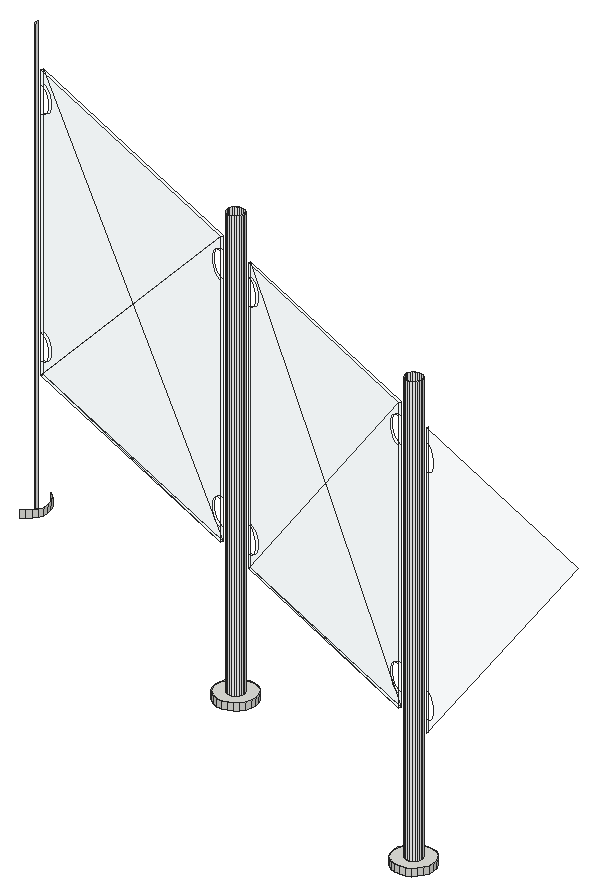
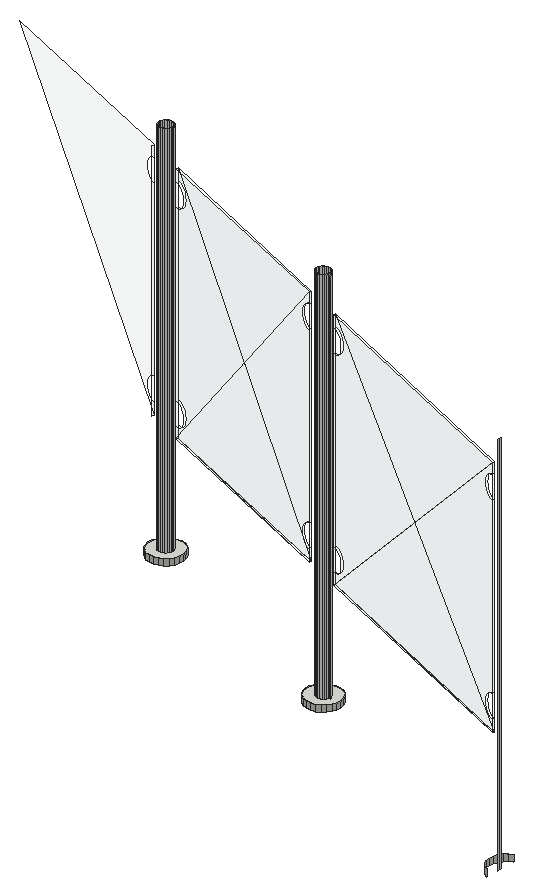
# SketchUp Ruby script. Lengths in inches.
U = 1.inch
M = Sketchup.active_model
def pt(a) = Geom::Point3d.new(a.map { |v| v * U })
def face(e, loops, mat)
  f = e.add_face(loops[0].map { |a| pt(a) })
  loops[1..].each { |l| e.add_face(l.map { |a| pt(a) }).erase! }
  f.material = f.back_material = mat if mat
  f
end
# faces: each face lists its corners as indices into pts; further lists are holes
def faces(e, pts, list, mat = nil) = list.each { |f| face(e, (f[0].is_a?(Array) ? f : [f]).map { |l| l.map { |i| pts[i] } }, mat) }
# xy, xz, yz: faces in a plane at the given z, y or x. An outline is a flat list of corners, or four numbers for a rectangle; further outlines are holes
def ring(l) = l.size == 4 ? [[l[0], l[1]], [l[2], l[1]], [l[2], l[3]], [l[0], l[3]]] : l.each_slice(2).to_a
def flat(e, list, mat, &to3) = list.each { |f| face(e, (f[0].is_a?(Array) ? f : [f]).map { |l| ring(l).map { |u, v| to3.(u, v) } }, mat) }
def xy(e, z, list, mat = nil) = flat(e, list, mat) { |x, y| [x, y, z] }
def xz(e, y, list, mat = nil) = flat(e, list, mat) { |x, z| [x, y, z] }
def yz(e, x, list, mat = nil) = flat(e, list, mat) { |y, z| [x, y, z] }
def lines(e, pts, list) = list.each { |a, b| e.add_line(pt(pts[a]), pt(pts[b])) }
# prism: a flat outline (further loops are holes) pulled along v
def prism(e, loops, v, mat = nil)
  f = face(e, loops, mat); d = Geom::Vector3d.new(v.map { |x| x * U })
  f.pushpull(f.normal.samedirection?(d) ? d.length : -d.length)
end
def box(e, o, s, mat = nil) = prism(e, [[o, [o[0] + s[0], o[1], o[2]], [o[0] + s[0], o[1] + s[1], o[2]], [o[0], o[1] + s[1], o[2]]]], [0, 0, s[2]], mat)
def at(x, y, z, deg = 0) = Geom::Transformation.translation(pt([x, y, z])) * Geom::Transformation.rotation(ORIGIN, Z_AXIS, deg.degrees)
def axes(o, x, y, z) = Geom::Transformation.new([*x, 0, *y, 0, *z, 0, *pt(o).to_a, 1])
def part(name) = M.definitions.add(name)
# library, detail: a bought-in or finely detailed component or shape, given as its bounding box
def library(name, o, s) = part(name).tap { |d| box(d.entities, o, s) }
def detail(e, o, s) = box(e.add_group.entities, o, s)
def put(e, d, t, mat = nil) = e.add_instance(d, t).tap { |i| i.material = mat if mat }
def group(e, t, mat = nil) = e.add_group.tap { |g| g.transformation = t; g.material = mat if mat }.entities
root = M.entities
M.materials.add("Glass_Safety_01").color = [204, 235, 244]
M.materials["Glass_Safety_01"].alpha = 0.1
M.materials.add("[Color_000]").color = [255, 255, 255]
xy(root,321.27,[[[723.14,584.81,723.54,584.89,723.91,585.07,724.22,585.35,724.44,585.69,724.57,586.08,724.6,586.49,724.51,586.89,724.33,587.26,724.06,587.57,723.71,587.8,723.32,587.92,722.91,587.95,722.51,587.87,722.14,587.68,721.83,587.41,721.61,587.07,721.59,587,721.48,586.68,721.45,586.27,721.54,585.86,721.72,585.5,721.99,585.1875,722.34,584.96,722.73,584.83],[723.07,585.75,722.91,585.76,722.75,585.8125,722.61,585.9,722.5,586.03,722.43,586.17,722.4,586.33,722.41,586.5,722.45,586.63,722.46,586.65,722.55,586.79,722.67,586.9,722.82,586.97,722.98,587.01,723.14,587,723.3,586.95,723.4375,586.85,723.55,586.73,723.62,586.58,723.65,586.42,723.64,586.26,723.6,586.13,723.59,586.1,723.5,585.97,723.38,585.86,723.23,585.78]],[724.46,585.75,724.57,586.08,724.6,586.49,724.51,586.89,724.33,587.26,724.06,587.57,723.71,587.8,723.32,587.92,722.91,587.95,722.51,587.87,722.14,587.68,721.83,587.41,721.61,587.07,721.59,587,722.45,586.63,722.46,586.65,722.55,586.79,722.67,586.9,722.82,586.97,722.98,587.01,723.14,587,723.3,586.95,723.4375,586.85,723.55,586.73,723.62,586.58,723.65,586.42,723.64,586.26,723.6,586.13],[723.6,586.13,723.64,586.26,723.65,586.42,723.62,586.58,723.55,586.73,723.4375,586.85,723.3,586.95,723.14,587,722.98,587.01,722.82,586.97,722.67,586.9,722.55,586.79,722.46,586.65,722.45,586.63],[[700.62,594.61,701.02,594.7,701.39,594.88,701.7,595.15,701.93,595.5,702.06,595.89,702.08,596.3,702,596.7,701.8125,597.07,701.54,597.375,701.2,597.6,700.81,597.73,700.4,597.76,699.99,597.67,699.625,597.49,699.32,597.22,699.09,596.87,699.07,596.8125,698.96,596.48,698.9375,596.07,699.02,595.67,699.2,595.3,699.48,594.99,699.82,594.77,700.21,594.64],[700.55,595.56,700.39,595.57,700.23,595.62,700.1,595.71,699.99,595.83,699.91,595.98,699.88,596.14,699.89,596.3,699.93,596.44,699.94,596.46,700.03,596.6,700.16,596.71,700.3,596.78,700.46,596.8125,700.63,596.8,700.78,596.75,700.92,596.66,701.03,596.54,701.1,596.39,701.14,596.23,701.13,596.07,701.08,595.93,701.08,595.91,700.98,595.77,700.86,595.66,700.71,595.59]],[701.95,595.56,702.06,595.89,702.08,596.3,702,596.7,701.8125,597.07,701.54,597.375,701.2,597.6,700.81,597.73,700.4,597.76,699.99,597.67,699.625,597.49,699.32,597.22,699.09,596.87,699.07,596.8125,699.93,596.44,699.94,596.46,700.03,596.6,700.16,596.71,700.3,596.78,700.46,596.8125,700.63,596.8,700.78,596.75,700.92,596.66,701.03,596.54,701.1,596.39,701.14,596.23,701.13,596.07,701.08,595.93],
  [701.08,595.93,701.13,596.07,701.14,596.23,701.1,596.39,701.03,596.54,700.92,596.66,700.78,596.75,700.63,596.8,700.46,596.8125,700.3,596.78,700.16,596.71,700.03,596.6,699.94,596.46,699.93,596.44]])
xy(root,321.27,[[723.07,585.75,723.23,585.78,723.38,585.86,723.5,585.97,723.59,586.1,723.6,586.13,722.45,586.63,722.41,586.5,722.4,586.33,722.43,586.17,722.5,586.03,722.61,585.9,722.75,585.8125,722.91,585.76],[700.55,595.56,700.71,595.59,700.86,595.66,700.98,595.77,701.08,595.91,701.08,595.93,699.93,596.44,699.89,596.3,699.88,596.14,699.91,595.98,699.99,595.83,700.1,595.71,700.23,595.62,700.39,595.57]],"[Color_000]")
xy(root,321.86,[[723.14,584.81,723.54,584.89,723.91,585.07,724.22,585.35,724.44,585.69,724.57,586.08,724.6,586.49,724.51,586.89,724.33,587.26,724.06,587.57,723.71,587.8,723.32,587.92,722.91,587.95,722.51,587.87,722.14,587.68,721.83,587.41,721.61,587.07,721.48,586.68,721.45,586.27,721.54,585.86,721.72,585.5,721.99,585.1875,722.34,584.96,722.73,584.83],[700.62,594.61,701.02,594.7,701.39,594.88,701.7,595.15,701.93,595.5,702.06,595.89,702.08,596.3,702,596.7,701.8125,597.07,701.54,597.375,701.2,597.6,700.81,597.73,700.4,597.76,699.99,597.67,699.625,597.49,699.32,597.22,699.09,596.87,698.96,596.48,698.9375,596.07,699.02,595.67,699.2,595.3,699.48,594.99,699.82,594.77,700.21,594.64]])
xy(root,331.9,[[721.33,587.01,702.27,595.31,702.35,595.49],[721.33,587.01,702.35,595.49,721.4,587.19],[698.79,596.83,676.04,606.74,676.12,606.92],[698.79,596.83,676.12,606.92,698.87,597.01]],"Glass_Safety_01")
p = [[722.34,584.96,321.27],[722.73,584.83,321.27],[722.73,584.83,321.86],[722.34,584.96,321.86],[723.14,584.81,321.27],[723.14,584.81,321.86],
  [723.54,584.89,321.27],[723.54,584.89,321.86],[723.91,585.07,321.27],[723.91,585.07,321.86],[721.99,585.1875,321.27],[721.99,585.1875,321.86],
  [724.22,585.35,321.27],[724.22,585.35,321.86],[721.72,585.5,321.27],[721.72,585.5,321.86],[724.44,585.69,321.27],[724.44,585.69,321.86],
  [721.54,585.86,321.27],[721.54,585.86,321.86],[724.46,585.75,321.27],[724.57,586.08,321.27],[724.57,586.08,321.86],[722.61,585.9,321.27],
  [722.75,585.8125,321.27],[722.75,585.8125,357.27],[722.61,585.9,357.27],[722.91,585.76,321.27],[722.91,585.76,357.27],[723.07,585.75,321.27],
  [723.07,585.75,357.27],[723.23,585.78,321.27],[723.23,585.78,357.27],[723.38,585.86,321.27],[723.38,585.86,357.27],[721.45,586.27,321.27],
  [721.45,586.27,321.86],[722.5,586.03,321.27],[722.5,586.03,357.27],[723.5,585.97,321.27],[723.5,585.97,357.27],[722.43,586.17,321.27],
  [722.43,586.17,357.27],[723.59,586.1,321.27],[723.59,586.1,357.27],[723.6,586.13,321.27],[723.64,586.26,321.27],[723.64,586.26,357.27],
  [724.6,586.49,321.27],[724.6,586.49,321.86],[722.4,586.33,321.27],[722.4,586.33,357.27],[721.48,586.68,321.27],[721.48,586.68,321.86],
  [722.41,586.5,321.27],[722.41,586.5,357.27],[723.65,586.42,321.27],[723.65,586.42,357.27],[723.62,586.58,321.27],[723.62,586.58,357.27],
  [722.46,586.65,321.27],[722.45,586.63,321.27],[722.46,586.65,357.27],[724.51,586.89,321.27],[724.51,586.89,321.86],[723.55,586.73,321.27],
  [723.55,586.73,357.27],[721.61,587.07,321.27],[721.59,587,321.27],[721.61,587.07,321.86],[722.55,586.79,321.27],[722.55,586.79,357.27],
  [723.4375,586.85,321.27],[723.4375,586.85,357.27],[722.67,586.9,321.27],[722.67,586.9,357.27],[722.82,586.97,321.27],[722.82,586.97,357.27],
  [723.3,586.95,321.27],[723.14,587,321.27],[723.14,587,357.27],[723.3,586.95,357.27],[724.33,587.26,321.27],[724.33,587.26,321.86],
  [722.98,587.01,321.27],[722.98,587.01,357.27],[721.83,587.41,321.27],[721.83,587.41,321.86],[724.06,587.57,321.27],[724.06,587.57,321.86],
  [722.14,587.68,321.27],[722.14,587.68,321.86],[723.71,587.8,321.27],[723.71,587.8,321.86],[722.51,587.87,321.27],[722.51,587.87,321.86],
  [723.32,587.92,321.27],[723.32,587.92,321.86],[722.91,587.95,321.27],[722.91,587.95,321.86],[699.82,594.77,321.27],[700.21,594.64,321.27],
  [700.21,594.64,321.86],[699.82,594.77,321.86],[700.62,594.61,321.27],[700.62,594.61,321.86],[701.02,594.7,321.27],[701.02,594.7,321.86],
  [701.39,594.88,321.27],[701.39,594.88,321.86],[699.48,594.99,321.27],[699.48,594.99,321.86],[701.7,595.15,321.27],[701.7,595.15,321.86],
  [699.2,595.3,321.27],[699.2,595.3,321.86],[701.93,595.5,321.27],[701.93,595.5,321.86],[699.02,595.67,321.27],[699.02,595.67,321.86],
  [701.95,595.56,321.27],[702.06,595.89,321.27],[702.06,595.89,321.86],[700.1,595.71,321.27],[700.23,595.62,321.27],[700.23,595.62,357.27],
  [700.1,595.71,357.27],[700.39,595.57,321.27],[700.39,595.57,357.27],[700.55,595.56,321.27],[700.55,595.56,357.27],[700.71,595.59,321.27],
  [700.71,595.59,357.27],[700.86,595.66,321.27],[700.86,595.66,357.27],[698.9375,596.07,321.27],[698.9375,596.07,321.86],[699.99,595.83,321.27],
  [699.99,595.83,357.27],[700.98,595.77,321.27],[700.98,595.77,357.27],[699.91,595.98,321.27],[699.91,595.98,357.27],[701.08,595.91,321.27],
  [701.08,595.91,357.27],[701.08,595.93,321.27],[701.13,596.07,321.27],[701.13,596.07,357.27],[702.08,596.3,321.27],[702.08,596.3,321.86],
  [699.88,596.14,321.27],[699.88,596.14,357.27],[698.96,596.48,321.27],[698.96,596.48,321.86],[699.89,596.3,321.27],[699.89,596.3,357.27],
  [701.14,596.23,321.27],[701.14,596.23,357.27],[701.1,596.39,321.27],[701.1,596.39,357.27],[699.94,596.46,321.27],[699.93,596.44,321.27],
  [699.94,596.46,357.27],[702,596.7,321.27],[702,596.7,321.86],[701.03,596.54,321.27],[701.03,596.54,357.27],[699.09,596.87,321.27],
  [699.07,596.8125,321.27],[699.09,596.87,321.86],[700.03,596.6,321.27],[700.03,596.6,357.27],[700.92,596.66,321.27],[700.92,596.66,357.27],
  [700.16,596.71,321.27],[700.16,596.71,357.27],[700.3,596.78,321.27],[700.3,596.78,357.27],[700.78,596.75,321.27],[700.78,596.75,357.27],
  [701.8125,597.07,321.27],[701.8125,597.07,321.86],[700.46,596.8125,321.27],[700.46,596.8125,357.27],[700.63,596.8,321.27],[700.63,596.8,357.27],
  [699.32,597.22,321.27],[699.32,597.22,321.86],[701.54,597.375,321.27],[701.54,597.375,321.86],[699.625,597.49,321.27],[699.625,597.49,321.86],
  [701.2,597.6,321.27],[701.2,597.6,321.86],[699.99,597.67,321.27],[699.99,597.67,321.86],[700.81,597.73,321.27],[700.81,597.73,321.86],
  [700.4,597.76,321.27],[700.4,597.76,321.86],[674.79,606.125,321.27],[675.15,606.31,321.27],[675.15,606.31,321.86],[674.79,606.125,321.86],
  [675.46,606.58,321.27],[675.46,606.58,321.86],[675.6875,606.92,321.27],[675.6875,606.92,321.86],[675.71,606.99,321.27],[675.82,607.3125,321.27],
  [675.82,607.3125,321.86],[675.84,607.72,321.27],[675.84,607.72,321.86],[674.89,607.49,321.27],[674.9,607.66,321.27],[674.9,607.66,357.27],
  [674.89,607.49,357.27],[674.87,607.82,321.27],[674.87,607.82,357.27],[675.76,608.13,321.27],[675.76,608.13,321.86],[675.58,608.49,321.27],
  [675.58,608.49,321.86],[675.3,608.8,321.27],[675.3,608.8,321.86],[674.96,609.03,321.27],[674.96,609.03,321.86],[724.79,585.5,351.28],
  [724.79,585.5,335.125],[725.04,585.39,335.09],[725.28,585.29,334.98],[725.48,585.2,334.8125],[725.63,585.13,334.59],[725.73,585.09,334.34],
  [725.76,585.08,334.0625],[725.73,585.09,333.79],[725.63,585.13,333.53],[725.48,585.2,333.3125],[725.28,585.29,333.14],[725.04,585.39,333.04],
  [724.79,585.5,333],[724.79,585.5,331.9],[744.03,577.12,354.51],[724.79,585.5,354.51],[724.79,585.5,353.41],[725.04,585.39,353.37],
  [725.28,585.29,353.27],[725.48,585.2,353.1],[725.63,585.13,352.88],[725.73,585.09,352.62],[725.76,585.08,352.35],[725.73,585.09,352.07],
  [725.63,585.13,351.81],[725.48,585.2,351.59],[725.28,585.29,351.43],[725.04,585.39,351.32],[724.87,585.68,331.9],[724.87,585.68,354.51],
  [724.87,585.68,353.41],[724.87,585.68,351.28],[724.87,585.68,335.125],[724.87,585.68,333],[702.27,595.31,351.28],[702.27,595.31,335.125],
  [702.53,595.2,335.09],[702.76,595.1,334.98],[702.96,595.01,334.8125],[703.12,594.94,334.59],[703.22,594.9,334.34],[703.25,594.88,334.0625],
  [703.22,594.9,333.79],[703.12,594.94,333.53],[702.96,595.01,333.3125],[702.76,595.1,333.14],[702.53,595.2,333.04],[702.27,595.31,333],
  [702.27,595.31,331.9],[721.33,587.01,354.51],[702.27,595.31,354.51],[702.27,595.31,353.41],[702.53,595.2,353.37],[702.76,595.1,353.27],
  [702.96,595.01,353.1],[703.12,594.94,352.88],[703.22,594.9,352.62],[703.25,594.88,352.35],[703.22,594.9,352.07],[703.12,594.94,351.81],
  [702.96,595.01,351.59],[702.76,595.1,351.43],[702.53,595.2,351.32],[721.33,587.01,331.9],[721.33,587.01,333],[721.18,587.07,333],
  [720.93,587.18,333.04],[720.69,587.29,333.14],[720.49,587.375,333.3125],[720.34,587.44,333.53],[720.24,587.48,333.79],[720.21,587.5,334.0625],
  [720.24,587.48,334.34],[720.34,587.44,334.59],[720.49,587.375,334.8125],[720.69,587.29,334.98],[720.93,587.18,335.09],[721.18,587.07,335.125],
  [721.33,587.01,335.125],[721.33,587.01,351.28],[721.18,587.07,351.28],[720.93,587.18,351.32],[720.69,587.29,351.43],[720.49,587.375,351.59],
  [720.34,587.44,351.81],[720.24,587.48,352.07],[720.21,587.5,352.35],[720.24,587.48,352.62],[720.34,587.44,352.88],[720.49,587.375,353.1],
  [720.69,587.29,353.27],[720.93,587.18,353.37],[721.18,587.07,353.41],[721.33,587.01,353.41],[721.4,587.19,331.9],[721.4,587.19,333],
  [721.4,587.19,335.125],[721.4,587.19,351.28],[721.4,587.19,353.41],[721.4,587.19,354.51],[702.35,595.49,331.9],[702.35,595.49,333],
  [702.61,595.38,333.04],[702.84,595.28,333.14],[703.04,595.1875,333.3125],[703.2,595.12,333.53],[703.29,595.08,333.79],[703.33,595.06,334.0625],
  [703.29,595.08,334.34],[703.2,595.12,334.59],[703.04,595.1875,334.8125],[702.84,595.28,334.98],[702.61,595.38,335.09],[702.35,595.49,335.125],
  [702.35,595.49,351.28],[702.61,595.38,351.32],[702.84,595.28,351.43],[703.04,595.1875,351.59],[703.2,595.12,351.81],[703.29,595.08,352.07],
  [703.33,595.06,352.35],[703.29,595.08,352.62],[703.2,595.12,352.88],[703.04,595.1875,353.1],[702.84,595.28,353.27],[702.61,595.38,353.37],
  [702.35,595.49,353.41],[702.35,595.49,354.51],[721.26,587.25,335.125],[721.01,587.36,335.09],[720.77,587.47,334.98],[720.57,587.55,334.8125],
  [720.42,587.62,334.59],[720.32,587.66,334.34],[720.28,587.68,334.0625],[720.32,587.66,333.79],[720.42,587.62,333.53],[720.57,587.55,333.3125],
  [720.77,587.47,333.14],[721.01,587.36,333.04],[721.26,587.25,333],[721.26,587.25,353.41],[721.01,587.36,353.37],[720.77,587.47,353.27],
  [720.57,587.55,353.1],[720.42,587.62,352.88],[720.32,587.66,352.62],[720.28,587.68,352.35],[720.32,587.66,352.07],[720.42,587.62,351.81],
  [720.57,587.55,351.59],[720.77,587.47,351.43],[721.01,587.36,351.32],[721.26,587.25,351.28],[676.04,606.74,351.28],[676.04,606.74,335.125],
  [676.29,606.625,335.09],[676.52,606.52,334.98],[676.73,606.44,334.8125],[676.88,606.37,334.59],[676.98,606.33,334.34],[677.01,606.3125,334.0625],
  [676.98,606.33,333.79],[676.88,606.37,333.53],[676.73,606.44,333.3125],[676.52,606.52,333.14],[676.29,606.625,333.04],[676.04,606.74,333],
  [676.04,606.74,331.9],[698.79,596.83,354.51],[676.04,606.74,354.51],[676.04,606.74,353.41],[676.29,606.625,353.37],[676.52,606.52,353.27],
  [676.73,606.44,353.1],[676.88,606.37,352.88],[676.98,606.33,352.62],[677.01,606.3125,352.35],[676.98,606.33,352.07],[676.88,606.37,351.81],
  [676.73,606.44,351.59],[676.52,606.52,351.43],[676.29,606.625,351.32],[698.79,596.83,331.9],[698.79,596.83,333],[698.66,596.88,333],
  [698.41,596.99,333.04],[698.18,597.09,333.14],[697.98,597.18,333.3125],[697.82,597.25,333.53],[697.72,597.29,333.79],[697.69,597.31,334.0625],
  [697.72,597.29,334.34],[697.82,597.25,334.59],[697.98,597.18,334.8125],[698.18,597.09,334.98],[698.41,596.99,335.09],[698.66,596.88,335.125],
  [698.79,596.83,335.125],[698.79,596.83,351.28],[698.66,596.88,351.28],[698.41,596.99,351.32],[698.18,597.09,351.43],[697.98,597.18,351.59],
  [697.82,597.25,351.81],[697.72,597.29,352.07],[697.69,597.31,352.35],[697.72,597.29,352.62],[697.82,597.25,352.88],[697.98,597.18,353.1],
  [698.18,597.09,353.27],[698.41,596.99,353.37],[698.66,596.88,353.41],[698.79,596.83,353.41],[698.87,597.01,331.9],[698.87,597.01,333],
  [698.87,597.01,335.125],[698.87,597.01,351.28],[698.87,597.01,353.41],[698.87,597.01,354.51],[676.12,606.92,331.9],[676.12,606.92,333],
  [676.37,606.81,333.04],[676.6,606.7,333.14],[676.81,606.62,333.3125],[676.96,606.55,333.53],[677.06,606.51,333.79],[677.09,606.49,334.0625],
  [677.06,606.51,334.34],[676.96,606.55,334.59],[676.81,606.62,334.8125],[676.6,606.7,334.98],[676.37,606.81,335.09],[676.12,606.92,335.125],
  [676.12,606.92,351.28],[676.37,606.81,351.32],[676.6,606.7,351.43],[676.81,606.62,351.59],[676.96,606.55,351.81],[677.06,606.51,352.07],
  [677.09,606.49,352.35],[677.06,606.51,352.62],[676.96,606.55,352.88],[676.81,606.62,353.1],[676.6,606.7,353.27],[676.37,606.81,353.37],
  [676.12,606.92,353.41],[676.12,606.92,354.51],[698.74,597.0625,335.125],[698.49,597.17,335.09],[698.26,597.27,334.98],[698.05,597.36,334.8125],
  [697.9,597.43,334.59],[697.8,597.47,334.34],[697.77,597.49,334.0625],[697.8,597.47,333.79],[697.9,597.43,333.53],[698.05,597.36,333.3125],
  [698.26,597.27,333.14],[698.49,597.17,333.04],[698.74,597.0625,333],[698.74,597.0625,353.41],[698.49,597.17,353.37],[698.26,597.27,353.27],
  [698.05,597.36,353.1],[697.9,597.43,352.88],[697.8,597.47,352.62],[697.77,597.49,352.35],[697.8,597.47,352.07],[697.9,597.43,351.81],
  [698.05,597.36,351.59],[698.26,597.27,351.43],[698.49,597.17,351.32],[698.74,597.0625,351.28]]
faces(root,p,[[0,1,2,3],[1,4,5,2],[4,6,7,5],[6,8,9,7],[10,0,3,11],[8,12,13,9],[14,10,11,15],[12,16,17,13],
  [18,14,15,19],[16,20,21,22,17],[35,18,19,36],[21,48,49,22],[52,35,36,53],[48,63,64,49],[67,68,52,53,69],[63,82,83,64],
  [86,67,69,87],[82,88,89,83],[90,86,87,91],[88,92,93,89],[94,90,91,95],[92,96,97,93],[98,94,95,99],[96,98,99,97],
  [100,101,102,103],[101,104,105,102],[104,106,107,105],[106,108,109,107],[110,100,103,111],[108,112,113,109],[114,110,111,115],[112,116,117,113],
  [118,114,115,119],[116,120,121,122,117],[135,118,119,136],[121,148,149,122],[152,135,136,153],[148,163,164,149],[167,168,152,153,169],[163,180,181,164],
  [186,167,169,187],[180,188,189,181],[190,186,187,191],[188,192,193,189],[194,190,191,195],[192,196,197,193],[198,194,195,199],[196,198,199,197],
  [200,201,202,203],[201,204,205,202],[204,206,207,205],[206,208,209,210,207],[209,211,212,210],[211,219,220,212],[219,221,222,220],[221,223,224,222],
  [223,225,226,224]])
faces(root,p,[[23,24,25,26],[24,27,28,25],[27,29,30,28],[29,31,32,30],[31,33,34,32],[37,23,26,38],[33,39,40,34],[41,37,38,42],
  [39,43,44,40],[43,45,46,47,44],[50,41,42,51],[54,50,51,55],[46,56,57,47],[56,58,59,57],[60,61,54,55,62],[58,65,66,59],
  [70,60,62,71],[65,72,73,66],[74,70,71,75],[76,74,75,77],[78,79,80,81],[72,78,81,73],[84,76,77,85],[79,84,85,80],
  [123,124,125,126],[124,127,128,125],[127,129,130,128],[129,131,132,130],[131,133,134,132],[137,123,126,138],[133,139,140,134],[141,137,138,142],
  [139,143,144,140],[143,145,146,147,144],[150,141,142,151],[154,150,151,155],[146,156,157,147],[156,158,159,157],[160,161,154,155,162],[158,165,166,159],
  [170,160,162,171],[165,172,173,166],[174,170,171,175],[176,174,175,177],[172,178,179,173],[182,176,177,183],[184,182,183,185],[178,184,185,179],
  [213,214,215,216],[214,217,218,215]],"[Color_000]")
faces(root,p,[[227,228,229,230,231,232,233,234,235,236,237,238,239,240,241,242,243,244,245,246,247,248,249,250,251,252,253,254,255],[256,241,240,228,227,244,243,257,258,259,260,261],[262,263,264,265,266,267,268,269,270,271,272,273,274,275,276,277,278,279,280,281,282,283,284,285,286,287,288,289,290],[291,292,293,294,295,296,297,298,299,300,301,302,303,304,305,306,307,308,309,310,311,312,313,314,315,316,317,318,319,320,321,277,276],[291,322,323,324,325,326,327,277,321,307,306,292],[328,329,330,331,332,333,334,335,336,337,338,339,340,341,342,343,344,345,346,347,348,349,350,351,352,353,354,355,322],[325,324,356,357,358,359,360,361,362,363,364,365,366,367,368,323,322,355,327,326,369,370,371,372,373,374,375,376,377,378,379,380,381],[328,276,275,263,262,279,278,355,354,342,341,329],
  [382,383,384,385,386,387,388,389,390,391,392,393,394,395,396,397,398,399,400,401,402,403,404,405,406,407,408,409,410],[411,412,413,414,415,416,417,418,419,420,421,422,423,424,425,426,427,428,429,430,431,432,433,434,435,436,437,438,439,440,441,397,396],[411,442,443,444,445,446,447,397,441,427,426,412],[448,449,450,451,452,453,454,455,456,457,458,459,460,461,462,463,464,465,466,467,468,469,470,471,472,473,474,475,442],[445,444,476,477,478,479,480,481,482,483,484,485,486,487,488,443,442,475,447,446,489,490,491,492,493,494,495,496,497,498,499,500,501],[448,396,395,383,382,399,398,475,474,462,461,449]],"Glass_Safety_01")
